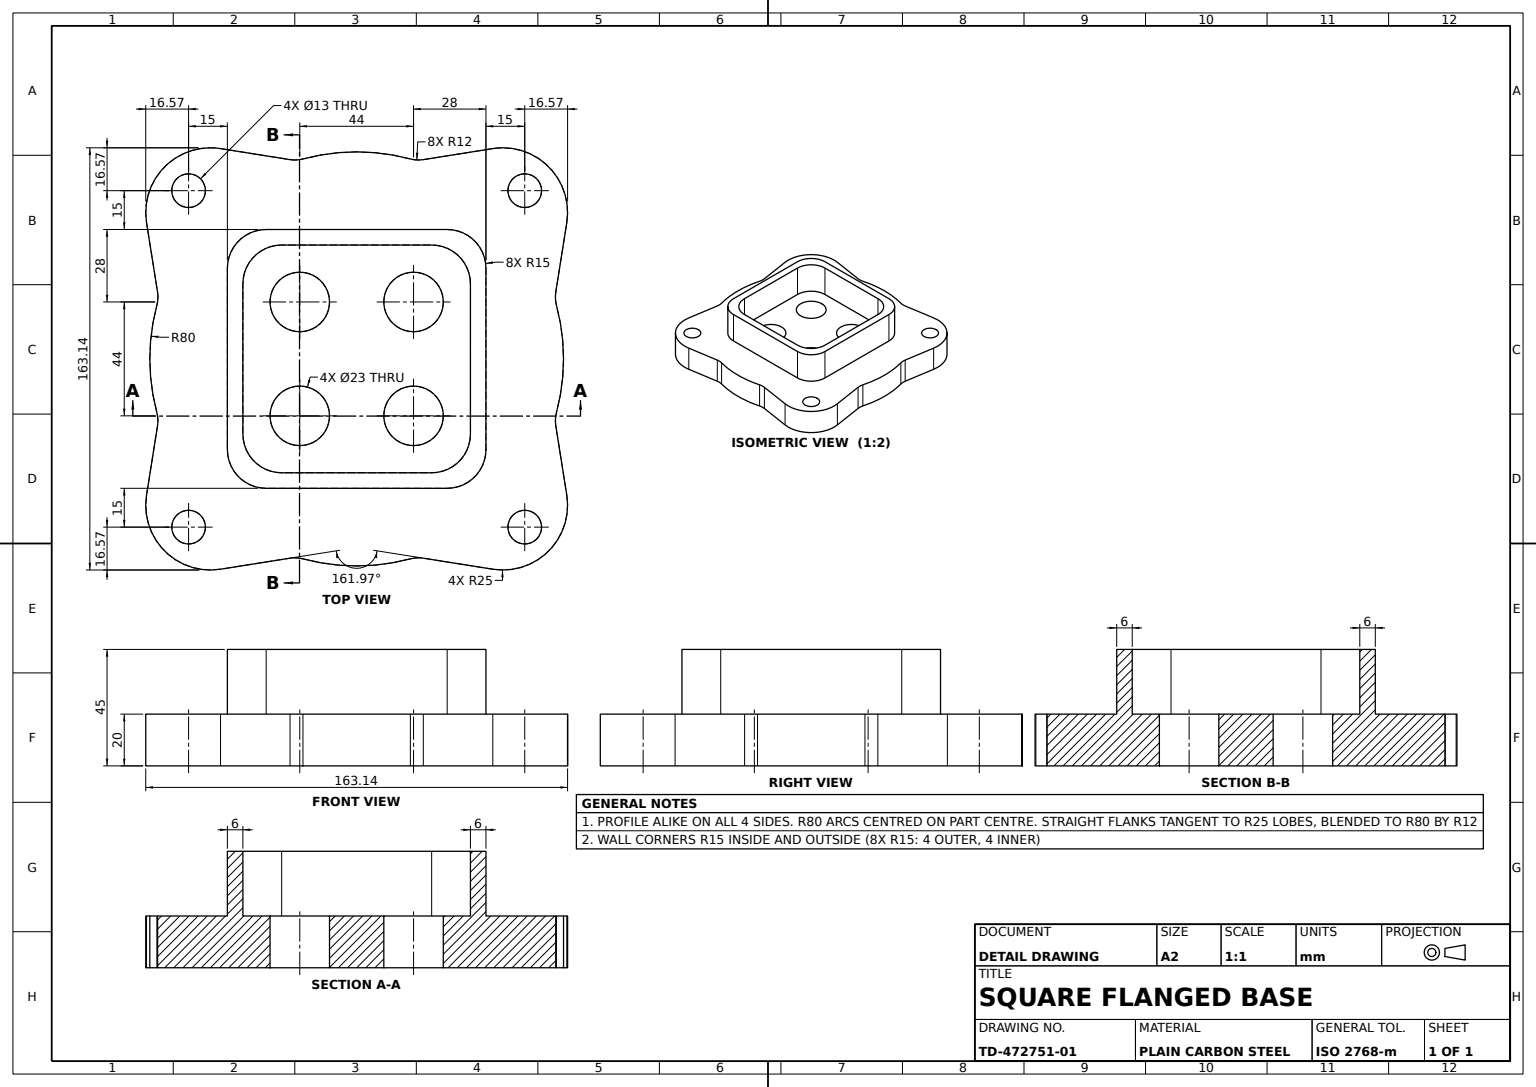
solid
v1 (65,20,71.5)
v2 (65,20,58.5)
e1 v1 v2 CIRCLE(AX(P(65,20,65),D(0,1,0),D(0,0,-1)),6.5)
v3 (65,0,58.5)
e2 v3 v2 LINE
v4 (65,0,71.5)
e3 v4 v3 CIRCLE(AX(P(65,0,65),D(0,1,0),D(0,0,1)),6.5)
e4 v4 v1 LINE
face CYL(AX(P(65,-5,65),D(0,1,0),D(0,0,1)),6.5) rev [e1 -e2 -e3 e4]
v5 (44,20,29)
v6 (44,20,-29)
e5 v5 v6 LINE
v7 (44,45,29)
e6 v7 v5 LINE
v8 (44,45,-29)
e7 v7 v8 LINE
e8 v8 v6 LINE
face PLANE(AX(P(44,45,1.641591),D(-1,0,0),D(0,0,1))) [-e5 -e6 e7 e8]
v9 (35,45,-50)
v10 (-35,45,-50)
e9 v9 v10 LINE
v11 (35,20,-50)
e10 v9 v11 LINE
v12 (-35,20,-50)
e11 v11 v12 LINE
e12 v10 v12 LINE
face PLANE(AX(P(-35,45,-50),D(0,0,1),D(1,0,0))) rev [-e9 e10 e11 -e12]
v13 (50,45,-35)
e13 v13 v9 CIRCLE(AX(P(35,45,-35),D(0,1,0),D(0,0,-1)),15)
v14 (50,20,-35)
e14 v13 v14 LINE
e15 v14 v11 CIRCLE(AX(P(35,20,-35),D(0,1,0),D(0,0,-1)),15)
face CYL(AX(P(35,45,-35),D(0,-1,0),D(0,0,-1)),15) [-e13 e14 e15 -e10]
v15 (-23.885958,0,76.845152)
v16 (-25.766692,0,76.99345)
e16 v15 v16 CIRCLE(AX(P(-23.885958,0,88.845152),D(0,1,0),D(0,0,1)),12)
v17 (-23.885958,20,76.845152)
e17 v17 v15 LINE
v18 (-25.766692,20,76.99345)
e18 v18 v17 CIRCLE(AX(P(-23.885958,20,88.845152),D(0,-1,0),D(0,0,1)),12)
e19 v16 v18 LINE
face CYL(AX(P(-23.885958,20,88.845152),D(0,-1,0),D(0,0,-1)),12) rev [-e16 -e17 -e18 -e19]
v19 (22,0,-33.5)
v20 (22,20,-33.5)
e20 v19 v20 LINE
v21 (22,20,-10.5)
e21 v20 v21 CIRCLE(AX(P(22,20,-22),D(0,1,0),D(0,0,-1)),11.5)
v22 (22,0,-10.5)
e22 v22 v21 LINE
e23 v19 v22 CIRCLE(AX(P(22,0,-22),D(0,1,0),D(0,0,1)),11.5)
face CYL(AX(P(22,-5,-22),D(0,1,0),D(0,0,1)),11.5) rev [e20 e21 -e22 -e23]
v23 (76.99345,20,-25.766692)
v24 (76.99345,0,-25.766692)
e24 v23 v24 LINE
v25 (77.256654,20,-20.770398)
e25 v25 v23 CIRCLE(AX(P(88.845152,20,-23.885958),D(0,-1,0),D(0,0,1)),12)
v26 (77.256654,0,-20.770398)
e26 v26 v25 LINE
e27 v24 v26 CIRCLE(AX(P(88.845152,0,-23.885958),D(0,1,0),D(0,0,1)),12)
face CYL(AX(P(88.845152,20,-23.885958),D(0,-1,0),D(0,0,-1)),12) rev [-e24 -e25 -e26 -e27]
v27 (20.770398,20,-77.256654)
v28 (20.770398,0,-77.256654)
e28 v27 v28 LINE
v29 (25.766692,20,-76.99345)
e29 v29 v27 CIRCLE(AX(P(23.885958,20,-88.845152),D(0,-1,0),D(0,0,1)),12)
v30 (25.766692,0,-76.99345)
e30 v30 v29 LINE
e31 v28 v30 CIRCLE(AX(P(23.885958,0,-88.845152),D(0,1,0),D(0,0,1)),12)
face CYL(AX(P(23.885958,20,-88.845152),D(0,-1,0),D(0,0,-1)),12) rev [-e28 -e29 -e30 -e31]
v31 (-52.650347,20,-81.259588)
v32 (-52.650347,0,-81.259588)
e32 v31 v32 LINE
v33 (-25.766692,20,-76.99345)
e33 v33 v31 LINE
v34 (-25.766692,0,-76.99345)
e34 v33 v34 LINE
e35 v34 v32 LINE
face PLANE(AX(P(-52.650347,20,-81.259588),D(-0.156727829,0,0.987641832),D(0.987641832,0,0.156727829))) rev [-e32 -e33 e34 e35]
e36 v3 v4 CIRCLE(AX(P(65,0,65),D(0,1,0),D(0,0,1)),6.5)
e37 v2 v1 CIRCLE(AX(P(65,20,65),D(0,1,0),D(0,0,-1)),6.5)
face CYL(AX(P(65,-5,65),D(0,1,0),D(0,0,1)),6.5) rev [-e4 -e36 e2 e37]
v35 (-65,0,58.5)
v36 (-65,0,71.5)
e38 v35 v36 CIRCLE(AX(P(-65,0,65),D(0,1,0),D(0,0,1)),6.5)
e39 v36 v35 CIRCLE(AX(P(-65,0,65),D(0,1,0),D(0,0,1)),6.5)
v37 (22,0,33.5)
v38 (22,0,10.5)
e40 v37 v38 CIRCLE(AX(P(22,0,22),D(0,1,0),D(0,0,1)),11.5)
e41 v38 v37 CIRCLE(AX(P(22,0,22),D(0,1,0),D(0,0,1)),11.5)
e42 v22 v19 CIRCLE(AX(P(22,0,-22),D(0,1,0),D(0,0,1)),11.5)
v39 (-65,0,-71.5)
v40 (-65,0,-58.5)
e43 v39 v40 CIRCLE(AX(P(-65,0,-65),D(0,1,0),D(0,0,1)),6.5)
e44 v40 v39 CIRCLE(AX(P(-65,0,-65),D(0,1,0),D(0,0,1)),6.5)
v41 (81.259588,0,-52.650347)
v42 (56.568542,0,-81.568542)
e45 v41 v42 CIRCLE(AX(P(56.568542,0,-56.568542),D(0,1,0),D(0,0,1)),25)
e46 v24 v41 LINE
v43 (77.256654,0,20.770398)
e47 v43 v26 CIRCLE(AX(P(0,0,0),D(0,1,0),D(0,0,1)),80)
v44 (76.99345,0,25.766692)
e48 v43 v44 CIRCLE(AX(P(88.845152,0,23.885958),D(0,1,0),D(0,0,1)),12)
v45 (81.259588,0,52.650347)
e49 v45 v44 LINE
v46 (52.650347,0,81.259588)
e50 v46 v45 CIRCLE(AX(P(56.568542,0,56.568542),D(0,1,0),D(0,0,1)),25)
v47 (25.766692,0,76.99345)
e51 v47 v46 LINE
v48 (23.885958,0,76.845152)
e52 v47 v48 CIRCLE(AX(P(23.885958,0,88.845152),D(0,1,0),D(0,0,1)),12)
v49 (20.770398,0,77.256654)
e53 v48 v49 CIRCLE(AX(P(23.885958,0,88.845152),D(0,1,0),D(0,0,1)),12)
v50 (-20.770398,0,77.256654)
e54 v50 v49 CIRCLE(AX(P(0,0,0),D(0,1,0),D(0,0,1)),80)
e55 v50 v15 CIRCLE(AX(P(-23.885958,0,88.845152),D(0,1,0),D(0,0,1)),12)
v51 (-52.650347,0,81.259588)
e56 v51 v16 LINE
v52 (-81.259588,0,52.650347)
e57 v52 v51 CIRCLE(AX(P(-56.568542,0,56.568542),D(0,1,0),D(0,0,1)),25)
v53 (-76.99345,0,25.766692)
e58 v53 v52 LINE
v54 (-77.256654,0,20.770398)
e59 v53 v54 CIRCLE(AX(P(-88.845152,0,23.885958),D(0,1,0),D(0,0,1)),12)
v55 (-77.256654,0,-20.770398)
e60 v55 v54 CIRCLE(AX(P(0,0,0),D(0,1,0),D(0,0,1)),80)
v56 (-76.99345,0,-25.766692)
e61 v55 v56 CIRCLE(AX(P(-88.845152,0,-23.885958),D(0,1,0),D(0,0,1)),12)
v57 (-81.259588,0,-52.650347)
e62 v57 v56 LINE
v58 (-56.568542,0,-81.568542)
e63 v58 v57 CIRCLE(AX(P(-56.568542,0,-56.568542),D(0,1,0),D(0,0,1)),25)
e64 v32 v58 CIRCLE(AX(P(-56.568542,0,-56.568542),D(0,1,0),D(0,0,1)),25)
v59 (-20.770398,0,-77.256654)
e65 v34 v59 CIRCLE(AX(P(-23.885958,0,-88.845152),D(0,1,0),D(0,0,1)),12)
v60 (0,0,-80)
e66 v60 v59 CIRCLE(AX(P(0,0,0),D(0,1,0),D(0,0,1)),80)
e67 v28 v60 CIRCLE(AX(P(0,0,0),D(0,1,0),D(0,0,1)),80)
v61 (52.650347,0,-81.259588)
e68 v61 v30 LINE
e69 v42 v61 CIRCLE(AX(P(56.568542,0,-56.568542),D(0,1,0),D(0,0,1)),25)
v62 (-22,0,-10.5)
v63 (-22,0,-33.5)
e70 v62 v63 CIRCLE(AX(P(-22,0,-22),D(0,1,0),D(0,0,1)),11.5)
e71 v63 v62 CIRCLE(AX(P(-22,0,-22),D(0,1,0),D(0,0,1)),11.5)
v64 (65,0,-71.5)
v65 (65,0,-58.5)
e72 v64 v65 CIRCLE(AX(P(65,0,-65),D(0,1,0),D(0,0,1)),6.5)
e73 v65 v64 CIRCLE(AX(P(65,0,-65),D(0,1,0),D(0,0,1)),6.5)
v66 (-22,0,33.5)
v67 (-22,0,10.5)
e74 v66 v67 CIRCLE(AX(P(-22,0,22),D(0,1,0),D(0,0,1)),11.5)
e75 v67 v66 CIRCLE(AX(P(-22,0,22),D(0,1,0),D(0,0,1)),11.5)
face PLANE(AX(P(0,0,0),D(0,1,0),D(0,0,1))) rev [e38 e39] [e40 e41] [e23 e42] [e43 e44] [-e45 -e46 e27 -e47 e48 -e49 -e50 -e51 e52 e53 -e54 e55 e16 -e56 -e57 -e58 e59 -e60 e61 -e62 -e63 -e64 -e35 e65 -e66 -e67 e31 -e68 -e69] [e70 e71] [e36 e3] [e72 e73] [e74 e75]
v68 (77.256654,20,20.770398)
e76 v68 v43 LINE
e77 v68 v25 CIRCLE(AX(P(0,20,0),D(0,1,0),D(0,0,1)),80)
face CYL(AX(P(0,20,0),D(0,-1,0),D(0,0,-1)),80) [e76 e47 e26 -e77]
v69 (81.259588,20,52.650347)
e78 v69 v45 LINE
v70 (76.99345,20,25.766692)
e79 v44 v70 LINE
e80 v69 v70 LINE
face PLANE(AX(P(81.259588,20,52.650347),D(-0.987641832,0,0.156727829),D(0.156727829,0,0.987641832))) rev [e78 e49 e79 -e80]
v71 (-44,20,29)
v72 (-29,20,44)
e81 v71 v72 CIRCLE(AX(P(-29,20,29),D(0,1,0),D(0,0,-1)),15)
v73 (-44,45,29)
e82 v73 v71 LINE
v74 (-29,45,44)
e83 v73 v74 CIRCLE(AX(P(-29,45,29),D(0,1,0),D(0,0,-1)),15)
e84 v74 v72 LINE
face CYL(AX(P(-29,45,29),D(0,-1,0),D(0,0,-1)),15) rev [-e81 -e82 e83 e84]
v75 (-56.568542,20,-81.568542)
e85 v31 v75 CIRCLE(AX(P(-56.568542,20,-56.568542),D(0,1,0),D(0,0,1)),25)
e86 v75 v58 LINE
face CYL(AX(P(-56.568542,20,-56.568542),D(0,-1,0),D(0,0,-1)),25) [-e85 e32 e64 -e86]
v76 (52.650347,20,-81.259588)
e87 v76 v29 LINE
e88 v76 v61 LINE
face PLANE(AX(P(52.650347,20,-81.259588),D(0.156727829,0,0.987641832),D(0.987641832,0,-0.156727829))) rev [e68 e30 -e87 e88]
v77 (29,45,-44)
e89 v8 v77 CIRCLE(AX(P(29,45,-29),D(0,1,0),D(0,0,-1)),15)
v78 (29,20,-44)
e90 v77 v78 LINE
e91 v6 v78 CIRCLE(AX(P(29,20,-29),D(0,1,0),D(0,0,-1)),15)
face CYL(AX(P(29,45,-29),D(0,-1,0),D(0,0,-1)),15) rev [e89 e90 -e91 -e8]
v79 (-22,20,-33.5)
e92 v63 v79 LINE
v80 (-22,20,-10.5)
e93 v62 v80 LINE
e94 v80 v79 CIRCLE(AX(P(-22,20,-22),D(0,1,0),D(0,0,1)),11.5)
face CYL(AX(P(-22,-5,-22),D(0,1,0),D(0,0,1)),11.5) rev [-e92 -e70 e93 e94]
v81 (23.885958,20,76.845152)
e95 v81 v48 LINE
v82 (20.770398,20,77.256654)
e96 v82 v81 CIRCLE(AX(P(23.885958,20,88.845152),D(0,-1,0),D(0,0,1)),12)
e97 v49 v82 LINE
face CYL(AX(P(23.885958,20,88.845152),D(0,-1,0),D(0,0,-1)),12) rev [-e95 -e96 -e97 -e53]
v83 (-65,20,58.5)
e98 v35 v83 LINE
v84 (-65,20,71.5)
e99 v83 v84 CIRCLE(AX(P(-65,20,65),D(0,1,0),D(0,0,1)),6.5)
e100 v36 v84 LINE
face CYL(AX(P(-65,-5,65),D(0,1,0),D(0,0,1)),6.5) rev [e98 e99 -e100 -e38]
v85 (50,45,35)
e101 v85 v13 LINE
v86 (-50,45,-35)
e102 v10 v86 CIRCLE(AX(P(-35,45,-35),D(0,1,0),D(0,0,-1)),15)
v87 (-50,45,35)
e103 v86 v87 LINE
v88 (-35,45,50)
e104 v87 v88 CIRCLE(AX(P(-35,45,35),D(0,1,0),D(0,0,-1)),15)
v89 (35,45,50)
e105 v88 v89 LINE
e106 v89 v85 CIRCLE(AX(P(35,45,35),D(0,1,0),D(0,0,-1)),15)
v90 (-29,45,-44)
e107 v77 v90 LINE
v91 (29,45,44)
e108 v91 v7 CIRCLE(AX(P(29,45,29),D(0,1,0),D(0,0,-1)),15)
e109 v74 v91 LINE
v92 (-44,45,-29)
e110 v92 v73 LINE
e111 v90 v92 CIRCLE(AX(P(-29,45,-29),D(0,1,0),D(0,0,1)),15)
face PLANE(AX(P(35,45,35),D(0,-1,0),D(0,0,-1))) rev [e101 e13 e9 e102 e103 e104 e105 e106] [-e107 -e89 -e7 -e108 -e109 -e83 -e110 -e111]
v93 (22,20,10.5)
e112 v38 v93 LINE
v94 (22,20,33.5)
e113 v37 v94 LINE
e114 v94 v93 CIRCLE(AX(P(22,20,22),D(0,1,0),D(0,0,1)),11.5)
face CYL(AX(P(22,-5,22),D(0,1,0),D(0,0,1)),11.5) rev [-e112 -e40 e113 e114]
v95 (-22,20,10.5)
e115 v67 v95 LINE
v96 (-22,20,33.5)
e116 v66 v96 LINE
e117 v96 v95 CIRCLE(AX(P(-22,20,22),D(0,1,0),D(0,0,-1)),11.5)
face CYL(AX(P(-22,-5,22),D(0,1,0),D(0,0,1)),11.5) rev [-e115 -e74 e116 e117]
e118 v21 v20 CIRCLE(AX(P(22,20,-22),D(0,1,0),D(0,0,-1)),11.5)
e119 v95 v96 CIRCLE(AX(P(-22,20,22),D(0,1,0),D(0,0,-1)),11.5)
e120 v79 v80 CIRCLE(AX(P(-22,20,-22),D(0,1,0),D(0,0,1)),11.5)
v97 (-29,20,-44)
e121 v78 v97 LINE
v98 (-44,20,-29)
e122 v97 v98 CIRCLE(AX(P(-29,20,-29),D(0,1,0),D(0,0,1)),15)
e123 v98 v71 LINE
v99 (29,20,44)
e124 v72 v99 LINE
e125 v99 v5 CIRCLE(AX(P(29,20,29),D(0,1,0),D(0,0,-1)),15)
e126 v93 v94 CIRCLE(AX(P(22,20,22),D(0,1,0),D(0,0,1)),11.5)
face PLANE(AX(P(0,20,0),D(0,1,0),D(0,0,1))) [-e21 -e118] [-e119 -e117] [-e94 -e120] [e91 e121 e122 e123 e81 e124 e125 e5] [-e126 -e114]
e127 v84 v83 CIRCLE(AX(P(-65,20,65),D(0,1,0),D(0,0,1)),6.5)
v100 (-65,20,-58.5)
v101 (-65,20,-71.5)
e128 v100 v101 CIRCLE(AX(P(-65,20,-65),D(0,1,0),D(0,0,-1)),6.5)
e129 v101 v100 CIRCLE(AX(P(-65,20,-65),D(0,1,0),D(0,0,-1)),6.5)
v102 (-50,20,-35)
e130 v12 v102 CIRCLE(AX(P(-35,20,-35),D(0,1,0),D(0,0,-1)),15)
v103 (50,20,35)
e131 v103 v14 LINE
v104 (35,20,50)
e132 v104 v103 CIRCLE(AX(P(35,20,35),D(0,1,0),D(0,0,-1)),15)
v105 (-35,20,50)
e133 v105 v104 LINE
v106 (-50,20,35)
e134 v106 v105 CIRCLE(AX(P(-35,20,35),D(0,1,0),D(0,0,-1)),15)
e135 v102 v106 LINE
v107 (65,20,-71.5)
v108 (65,20,-58.5)
e136 v107 v108 CIRCLE(AX(P(65,20,-65),D(0,1,0),D(0,0,1)),6.5)
e137 v108 v107 CIRCLE(AX(P(65,20,-65),D(0,1,0),D(0,0,1)),6.5)
v109 (0,20,-80)
e138 v27 v109 CIRCLE(AX(P(0,20,0),D(0,1,0),D(0,0,1)),80)
v110 (-20.770398,20,-77.256654)
e139 v109 v110 CIRCLE(AX(P(0,20,0),D(0,1,0),D(0,0,1)),80)
e140 v110 v33 CIRCLE(AX(P(-23.885958,20,-88.845152),D(0,-1,0),D(0,0,1)),12)
v111 (-81.259588,20,-52.650347)
e141 v75 v111 CIRCLE(AX(P(-56.568542,20,-56.568542),D(0,1,0),D(0,0,1)),25)
v112 (-76.99345,20,-25.766692)
e142 v111 v112 LINE
v113 (-77.256654,20,-20.770398)
e143 v112 v113 CIRCLE(AX(P(-88.845152,20,-23.885958),D(0,-1,0),D(0,0,1)),12)
v114 (-77.256654,20,20.770398)
e144 v113 v114 CIRCLE(AX(P(0,20,0),D(0,1,0),D(0,0,1)),80)
v115 (-76.99345,20,25.766692)
e145 v114 v115 CIRCLE(AX(P(-88.845152,20,23.885958),D(0,-1,0),D(0,0,1)),12)
v116 (-81.259588,20,52.650347)
e146 v115 v116 LINE
v117 (-52.650347,20,81.259588)
e147 v116 v117 CIRCLE(AX(P(-56.568542,20,56.568542),D(0,1,0),D(0,0,1)),25)
e148 v117 v18 LINE
v118 (-20.770398,20,77.256654)
e149 v17 v118 CIRCLE(AX(P(-23.885958,20,88.845152),D(0,-1,0),D(0,0,1)),12)
e150 v118 v82 CIRCLE(AX(P(0,20,0),D(0,1,0),D(0,0,1)),80)
v119 (25.766692,20,76.99345)
e151 v81 v119 CIRCLE(AX(P(23.885958,20,88.845152),D(0,-1,0),D(0,0,1)),12)
v120 (52.650347,20,81.259588)
e152 v119 v120 LINE
e153 v120 v69 CIRCLE(AX(P(56.568542,20,56.568542),D(0,1,0),D(0,0,1)),25)
e154 v70 v68 CIRCLE(AX(P(88.845152,20,23.885958),D(0,-1,0),D(0,0,1)),12)
v121 (81.259588,20,-52.650347)
e155 v23 v121 LINE
v122 (56.568542,20,-81.568542)
e156 v121 v122 CIRCLE(AX(P(56.568542,20,-56.568542),D(0,1,0),D(0,0,1)),25)
e157 v122 v76 CIRCLE(AX(P(56.568542,20,-56.568542),D(0,1,0),D(0,0,1)),25)
face PLANE(AX(P(0,20,0),D(0,1,0),D(0,0,1))) [-e127 -e99] [-e128 -e129] [-e130 -e11 -e15 -e131 -e132 -e133 -e134 -e135] [-e136 -e137] [-e37 -e1] [e138 e139 e140 e33 e85 e141 e142 e143 e144 e145 e146 e147 e148 e18 e149 e150 e96 e151 e152 e153 e80 e154 e77 e25 e155 e156 e157 e87 e29]
e158 v119 v47 LINE
face CYL(AX(P(23.885958,20,88.845152),D(0,-1,0),D(0,0,-1)),12) rev [-e151 e95 -e52 -e158]
e159 v89 v104 LINE
e160 v88 v105 LINE
face PLANE(AX(P(35,45,50),D(0,0,-1),D(-1,0,0))) rev [e133 -e159 -e105 e160]
e161 v90 v97 LINE
e162 v92 v98 LINE
face CYL(AX(P(-29,45,-29),D(0,-1,0),D(0,0,-1)),15) rev [-e122 -e161 e111 e162]
face CYL(AX(P(-22,-5,22),D(0,1,0),D(0,0,1)),11.5) rev [e119 -e116 -e75 e115]
e163 v59 v110 LINE
face CYL(AX(P(-23.885958,20,-88.845152),D(0,-1,0),D(0,0,-1)),12) rev [-e65 -e34 -e140 -e163]
e164 v118 v50 LINE
face CYL(AX(P(0,20,0),D(0,-1,0),D(0,0,-1)),80) [-e150 e164 e54 e97]
e165 v120 v46 LINE
face PLANE(AX(P(52.650347,20,81.259588),D(0.156727829,0,-0.987641832),D(-0.987641832,0,-0.156727829))) rev [-e165 -e152 e158 e51]
e166 v56 v112 LINE
e167 v113 v55 LINE
face CYL(AX(P(-88.845152,20,-23.885958),D(0,-1,0),D(0,0,-1)),12) rev [-e143 -e166 -e61 -e167]
face CYL(AX(P(-65,-5,65),D(0,1,0),D(0,0,1)),6.5) rev [-e39 e100 e127 -e98]
e168 v122 v42 LINE
face CYL(AX(P(56.568542,20,-56.568542),D(0,-1,0),D(0,0,-1)),25) [e69 -e88 -e157 e168]
face CYL(AX(P(-23.885958,20,88.845152),D(0,-1,0),D(0,0,-1)),12) rev [-e55 -e164 -e149 e17]
e169 v109 v60 LINE
face CYL(AX(P(0,20,0),D(0,-1,0),D(0,0,-1)),80) [-e169 -e138 e28 e67]
face CYL(AX(P(88.845152,20,23.885958),D(0,-1,0),D(0,0,-1)),12) rev [-e76 -e154 -e79 -e48]
e170 v121 v41 LINE
face CYL(AX(P(56.568542,20,-56.568542),D(0,-1,0),D(0,0,-1)),25) [e45 -e168 -e156 e170]
face PLANE(AX(P(81.259588,20,-52.650347),D(-0.987641832,0,-0.156727829),D(-0.156727829,0,0.987641832))) rev [-e170 -e155 e24 e46]
e171 v111 v57 LINE
face CYL(AX(P(-56.568542,20,-56.568542),D(0,-1,0),D(0,0,-1)),25) [-e141 e86 e63 -e171]
e172 v54 v114 LINE
face CYL(AX(P(0,20,0),D(0,-1,0),D(0,0,-1)),80) [e172 -e144 e167 e60]
face PLANE(AX(P(-29,45,-44),D(0,0,1),D(1,0,0))) [-e90 e107 e161 -e121]
e173 v40 v100 LINE
e174 v39 v101 LINE
face CYL(AX(P(-65,-5,-65),D(0,1,0),D(0,0,1)),6.5) rev [-e44 e173 e128 -e174]
face CYL(AX(P(56.568542,20,56.568542),D(0,-1,0),D(0,0,-1)),25) [e165 e50 -e78 -e153]
face CYL(AX(P(-22,-5,-22),D(0,1,0),D(0,0,1)),11.5) rev [-e93 -e71 e92 e120]
e175 v87 v106 LINE
face CYL(AX(P(-35,45,35),D(0,-1,0),D(0,0,-1)),15) [-e104 e175 e134 -e160]
e176 v116 v52 LINE
e177 v115 v53 LINE
face PLANE(AX(P(-81.259588,20,52.650347),D(0.987641832,0,0.156727829),D(0.156727829,0,-0.987641832))) rev [e58 -e176 -e146 e177]
e178 v85 v103 LINE
face CYL(AX(P(35,45,35),D(0,-1,0),D(0,0,-1)),15) [e132 -e178 -e106 e159]
face PLANE(AX(P(-44,45,29),D(1,0,0),D(0,0,-1))) [e82 -e123 -e162 e110]
face CYL(AX(P(0,20,0),D(0,-1,0),D(0,0,-1)),80) [e163 -e139 e169 e66]
face CYL(AX(P(-65,-5,-65),D(0,1,0),D(0,0,1)),6.5) rev [e129 -e173 -e43 e174]
e179 v91 v99 LINE
face PLANE(AX(P(29,45,44),D(0,0,-1),D(-1,0,0))) [e179 -e124 -e84 e109]
e180 v64 v107 LINE
e181 v65 v108 LINE
face CYL(AX(P(65,-5,-65),D(0,1,0),D(0,0,1)),6.5) rev [-e180 -e73 e181 e137]
e182 v86 v102 LINE
face PLANE(AX(P(-50,45,35),D(1,0,0),D(0,0,-1))) rev [e182 e135 -e175 -e103]
face CYL(AX(P(22,-5,22),D(0,1,0),D(0,0,1)),11.5) rev [e112 e126 -e113 -e41]
e183 v117 v51 LINE
face CYL(AX(P(-56.568542,20,56.568542),D(0,-1,0),D(0,0,-1)),25) [e176 e57 -e183 -e147]
face PLANE(AX(P(50,45,1.641591),D(-1,0,0),D(0,0,1))) rev [e131 -e14 -e101 e178]
face PLANE(AX(P(-81.259588,20,-52.650347),D(0.987641832,0,-0.156727829),D(-0.156727829,0,-0.987641832))) rev [e166 -e142 e171 e62]
face CYL(AX(P(-35,45,-35),D(0,-1,0),D(0,0,-1)),15) [e130 -e182 -e102 e12]
face CYL(AX(P(29,45,29),D(0,-1,0),D(0,0,-1)),15) rev [-e179 e108 e6 -e125]
face CYL(AX(P(-88.845152,20,23.885958),D(0,-1,0),D(0,0,-1)),12) rev [-e145 -e172 -e59 -e177]
face PLANE(AX(P(-52.650347,20,81.259588),D(-0.156727829,0,-0.987641832),D(-0.987641832,0,0.156727829))) rev [e56 e19 -e148 e183]
face CYL(AX(P(65,-5,-65),D(0,1,0),D(0,0,1)),6.5) rev [-e72 e180 e136 -e181]
face CYL(AX(P(22,-5,-22),D(0,1,0),D(0,0,1)),11.5) rev [-e20 -e42 e22 e118]
